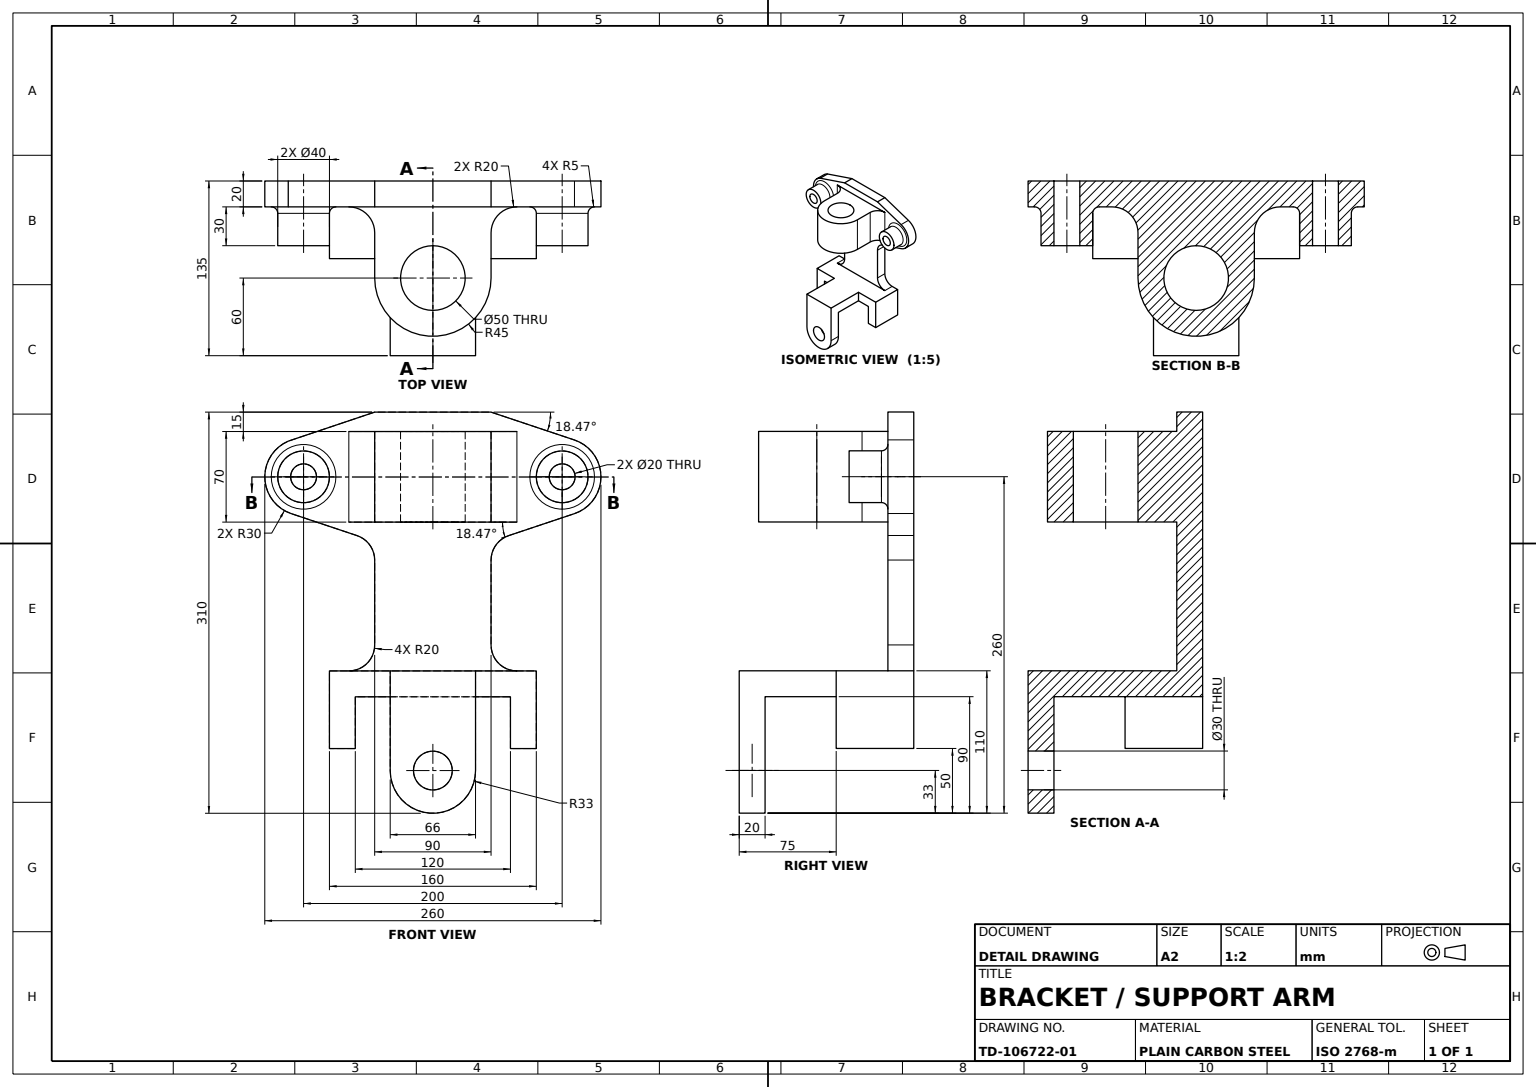
solid
v1 (-45,260,0)
v2 (-111.862968,237.554854,0)
e1 v1 v2 LINE
v3 (-111.862968,237.554854,20)
e2 v2 v3 LINE
v4 (-45,260,20)
e3 v4 v3 LINE
e4 v1 v4 LINE
face PLANE(AX(P(-45,260,0),D(-0.318236717,0.948011283,0),D(-0.948011283,-0.318236717,0))) [e1 e2 -e3 -e4]
v5 (109.504259,181.545316,20)
v6 (130,210,20)
e5 v5 v6 CIRCLE(AX(P(100,210,20),D(0,0,1),D(1,0,0)),30)
v7 (109.504259,181.545316,0)
e6 v7 v5 LINE
v8 (130,210,0)
e7 v7 v8 CIRCLE(AX(P(100,210,0),D(0,0,1),D(1,0,0)),30)
e8 v8 v6 LINE
face CYL(AX(P(100,210,0),D(0,0,1),D(1,0,0)),30) [-e5 -e6 e7 e8]
v9 (-75,210,20)
v10 (-125,210,20)
e9 v9 v10 CIRCLE(AX(P(-100,210,20),D(0,0,-1),D(-1,0,0)),25)
e10 v10 v9 CIRCLE(AX(P(-100,210,20),D(0,0,-1),D(-1,0,0)),25)
v11 (65,245,20)
v12 (-65,245,20)
e11 v11 v12 LINE
v13 (65,175,20)
e12 v11 v13 LINE
v14 (-65,175,20)
e13 v13 v14 LINE
e14 v14 v12 LINE
v15 (125,210,20)
v16 (75,210,20)
e15 v15 v16 CIRCLE(AX(P(100,210,20),D(0,0,-1),D(-1,0,0)),25)
e16 v16 v15 CIRCLE(AX(P(100,210,20),D(0,0,-1),D(-1,0,0)),25)
v17 (-58.663828,164.563908,20)
v18 (-45,145.594118,20)
e17 v17 v18 CIRCLE(AX(P(-65,145.594118,20),D(0,0,-1),D(-1,0,0)),20)
v19 (-45,80,20)
e18 v19 v18 LINE
v20 (-65,60,20)
e19 v19 v20 CIRCLE(AX(P(-65,80,20),D(0,0,-1),D(-1,0,0)),20)
v21 (65,60,20)
e20 v21 v20 LINE
v22 (45,80,20)
e21 v21 v22 CIRCLE(AX(P(65,80,20),D(0,0,-1),D(-1,0,0)),20)
v23 (45,145.594118,20)
e22 v23 v22 LINE
v24 (58.663828,164.563908,20)
e23 v23 v24 CIRCLE(AX(P(65,145.594118,20),D(0,0,-1),D(-1,0,0)),20)
e24 v24 v5 LINE
v25 (109.504259,238.454684,20)
e25 v6 v25 CIRCLE(AX(P(100,210,20),D(0,0,1),D(1,0,0)),30)
v26 (45,260,20)
e26 v25 v26 LINE
e27 v26 v4 LINE
v27 (-109.504259,181.545316,20)
e28 v3 v27 CIRCLE(AX(P(-100,210,20),D(0,0,1),D(1,0,0)),30)
e29 v27 v17 LINE
face PLANE(AX(P(0,0,20),D(0,0,-1),D(-1,0,0))) rev [e9 e10] [-e11 e12 e13 e14] [e15 e16] [e17 -e18 e19 -e20 e21 -e22 e23 e24 e5 e25 e26 e27 e3 e28 e29]
v28 (45,260,0)
e30 v28 v26 LINE
e31 v28 v1 LINE
face PLANE(AX(P(0,260,0),D(0,1,0),D(0,0,1))) [-e27 -e30 e31 e4]
v29 (-109.504259,181.545316,0)
e32 v29 v27 LINE
v30 (-58.663828,164.563908,0)
e33 v29 v30 LINE
e34 v30 v17 LINE
face PLANE(AX(P(-109.504259,181.545316,0),D(-0.31680862,-0.948489482,0),D(0.948489482,-0.31680862,0))) [-e29 -e32 e33 e34]
v31 (-120,210,25)
v32 (-80,210,25)
e35 v31 v32 CIRCLE(AX(P(-100,210,25),D(0,0,1),D(-1,0,0)),20)
v33 (-80,210,50)
e36 v33 v32 LINE
v34 (-120,210,50)
e37 v34 v33 CIRCLE(AX(P(-100,210,50),D(0,0,1),D(1,0,0)),20)
e38 v34 v31 LINE
face CYL(AX(P(-100,210,50),D(0,0,-1),D(-1,0,0)),20) [e35 -e36 -e37 e38]
v35 (90,210,50)
v36 (110,210,50)
e39 v35 v36 CIRCLE(AX(P(100,210,50),D(0,0,1),D(1,0,0)),10)
v37 (110,210,0)
e40 v37 v36 LINE
v38 (90,210,0)
e41 v38 v37 CIRCLE(AX(P(100,210,0),D(0,0,1),D(1,0,0)),10)
e42 v38 v35 LINE
face CYL(AX(P(100,210,-32),D(0,0,1),D(1,0,0)),10) rev [e39 -e40 -e41 e42]
v39 (15,-17,135)
v40 (-15,-17,135)
e43 v39 v40 CIRCLE(AX(P(0,-17,135),D(0,0,1),D(1,0,0)),15)
v41 (-15,-17,115)
e44 v41 v40 LINE
v42 (15,-17,115)
e45 v42 v41 CIRCLE(AX(P(0,-17,115),D(0,0,1),D(1,0,0)),15)
e46 v42 v39 LINE
face CYL(AX(P(0,-17,-80),D(0,0,1),D(1,0,0)),15) rev [e43 -e44 -e45 e46]
v43 (-60,40,60)
v44 (-60,40,0)
e47 v43 v44 LINE
v45 (-60,0,60)
e48 v45 v43 LINE
v46 (-60,0,0)
e49 v45 v46 LINE
e50 v46 v44 LINE
face PLANE(AX(P(-60,0,60),D(-1,0,0),D(0,0,1))) rev [-e47 -e48 e49 e50]
v47 (60,0,60)
v48 (80,0,60)
e51 v47 v48 LINE
v49 (60,0,0)
e52 v47 v49 LINE
v50 (80,0,0)
e53 v49 v50 LINE
e54 v48 v50 LINE
face PLANE(AX(P(60,0,60),D(0,1,0),D(0,0,1))) rev [-e51 e52 e53 -e54]
v51 (-33,-17,115)
v52 (-33,-17,135)
e55 v51 v52 LINE
v53 (33,-17,115)
e56 v51 v53 CIRCLE(AX(P(0,-17,115),D(0,0,1),D(1,0,0)),33)
v54 (33,-17,135)
e57 v53 v54 LINE
e58 v52 v54 CIRCLE(AX(P(0,-17,135),D(0,0,1),D(1,0,0)),33)
face CYL(AX(P(0,-17,115),D(0,0,1),D(1,0,0)),33) [-e55 e56 e57 -e58]
v55 (-90,210,0)
v56 (-90,210,50)
e59 v55 v56 LINE
v57 (-110,210,0)
e60 v57 v55 CIRCLE(AX(P(-100,210,0),D(0,0,1),D(1,0,0)),10)
v58 (-110,210,50)
e61 v57 v58 LINE
e62 v58 v56 CIRCLE(AX(P(-100,210,50),D(0,0,1),D(1,0,0)),10)
face CYL(AX(P(-100,210,-32),D(0,0,1),D(1,0,0)),10) rev [-e59 -e60 e61 e62]
e63 v32 v31 CIRCLE(AX(P(-100,210,25),D(0,0,1),D(-1,0,0)),20)
e64 v33 v34 CIRCLE(AX(P(-100,210,50),D(0,0,1),D(1,0,0)),20)
face CYL(AX(P(-100,210,50),D(0,0,-1),D(-1,0,0)),20) [e63 -e38 -e64 e36]
v59 (-80,0,60)
e65 v59 v45 LINE
v60 (-80,0,0)
e66 v59 v60 LINE
e67 v60 v46 LINE
face PLANE(AX(P(-80,0,60),D(0,1,0),D(0,0,1))) rev [-e65 e66 e67 -e49]
e68 v41 v42 CIRCLE(AX(P(0,-17,115),D(0,0,1),D(1,0,0)),15)
e69 v40 v39 CIRCLE(AX(P(0,-17,135),D(0,0,1),D(1,0,0)),15)
face CYL(AX(P(0,-17,-80),D(0,0,1),D(1,0,0)),15) rev [-e46 -e68 e44 e69]
v61 (60,40,60)
e70 v61 v47 LINE
v62 (60,40,0)
e71 v61 v62 LINE
e72 v62 v49 LINE
face PLANE(AX(P(60,40,60),D(1,0,0),D(0,0,-1))) rev [-e70 e71 e72 -e52]
v63 (45,80,0)
e73 v22 v63 LINE
v64 (45,145.594118,0)
e74 v64 v63 LINE
e75 v64 v23 LINE
face PLANE(AX(P(45,160,20),D(1,0,0),D(0,0,-1))) [e73 -e74 e75 e22]
v65 (65,60,0)
e76 v65 v21 LINE
e77 v63 v65 CIRCLE(AX(P(65,80,0),D(0,0,1),D(1,0,0)),20)
face CYL(AX(P(65,80,20),D(0,0,-1),D(-1,0,0)),20) rev [-e73 -e21 -e76 -e77]
v66 (-45,245,75)
v67 (-45,175,75)
e78 v66 v67 LINE
v68 (45,175,75)
e79 v67 v68 CIRCLE(AX(P(0,175,75),D(0,1,0),D(0,0,1)),45)
v69 (45,245,75)
e80 v69 v68 LINE
e81 v66 v69 CIRCLE(AX(P(0,245,75),D(0,1,0),D(0,0,1)),45)
face CYL(AX(P(0,245,75),D(0,-1,0),D(0,0,-1)),45) [e78 e79 -e80 -e81]
v70 (0,175,100)
v71 (0,245,100)
e82 v70 v71 LINE
v72 (0,175,50)
e83 v72 v70 CIRCLE(AX(P(0,175,75),D(0,1,0),D(0,0,1)),25)
v73 (0,245,50)
e84 v72 v73 LINE
e85 v73 v71 CIRCLE(AX(P(0,245,75),D(0,1,0),D(0,0,1)),25)
face CYL(AX(P(0,163,75),D(0,1,0),D(0,0,1)),25) rev [-e82 -e83 e84 e85]
e86 v56 v58 CIRCLE(AX(P(-100,210,50),D(0,0,1),D(1,0,0)),10)
e87 v55 v57 CIRCLE(AX(P(-100,210,0),D(0,0,1),D(1,0,0)),10)
face CYL(AX(P(-100,210,-32),D(0,0,1),D(1,0,0)),10) rev [e86 -e61 -e87 e59]
v74 (-45,145.594118,0)
e88 v18 v74 LINE
v75 (-45,80,0)
e89 v75 v74 LINE
e90 v75 v19 LINE
face PLANE(AX(P(-45,60,20),D(-1,0,0),D(0,0,1))) [e18 e88 -e89 e90]
e91 v70 v72 CIRCLE(AX(P(0,175,75),D(0,1,0),D(0,0,1)),25)
e92 v71 v73 CIRCLE(AX(P(0,245,75),D(0,1,0),D(0,0,1)),25)
face CYL(AX(P(0,163,75),D(0,1,0),D(0,0,1)),25) rev [-e84 -e91 e82 e92]
e93 v9 v32 CIRCLE(AX(P(-75,210,25),D(0,1,0),D(-1,0,0)),5)
e94 v10 v31 CIRCLE(AX(P(-125,210,25),D(0,-1,0),D(0,0,-1)),5)
face TORUS(AX(P(-100,210,25),D(0,0,-1),D(-1,0,0)),25,5) rev [-e93 -e10 e94 -e63]
v76 (-65,60,0)
e95 v76 v75 CIRCLE(AX(P(-65,80,0),D(0,0,1),D(1,0,0)),20)
e96 v20 v76 LINE
face CYL(AX(P(-65,80,60),D(0,0,-1),D(-1,0,0)),20) rev [-e90 -e95 -e96 -e19]
v77 (33,40,60)
e97 v77 v61 LINE
v78 (33,40,115)
e98 v78 v77 LINE
v79 (-33,40,115)
e99 v78 v79 LINE
v80 (-33,40,60)
e100 v80 v79 LINE
e101 v43 v80 LINE
e102 v44 v62 LINE
face PLANE(AX(P(-60,40,60),D(0,1,0),D(0,0,1))) rev [-e97 -e98 e99 -e100 -e101 e47 e102 -e71]
v81 (45,245,40)
e103 v69 v81 LINE
v82 (45,175,40)
e104 v68 v82 LINE
e105 v82 v81 LINE
face PLANE(AX(P(45,245,20),D(-1,0,0),D(0,0,1))) rev [-e103 e80 e104 e105]
face TORUS(AX(P(-100,210,25),D(0,0,-1),D(-1,0,0)),25,5) rev [-e9 e93 -e35 -e94]
v83 (120,210,25)
e106 v15 v83 CIRCLE(AX(P(125,210,25),D(0,1,0),D(-1,0,0)),5)
v84 (80,210,25)
e107 v84 v83 CIRCLE(AX(P(100,210,25),D(0,0,1),D(-1,0,0)),20)
e108 v16 v84 CIRCLE(AX(P(75,210,25),D(0,-1,0),D(0,0,-1)),5)
face TORUS(AX(P(100,210,25),D(0,0,-1),D(-1,0,0)),25,5) rev [e106 -e107 -e108 -e15]
v85 (-80,60,60)
e109 v85 v59 LINE
v86 (-80,60,0)
e110 v85 v86 LINE
e111 v86 v60 LINE
face PLANE(AX(P(-80,60,60),D(1,0,0),D(0,0,-1))) rev [-e109 e110 e111 -e66]
e112 v81 v11 CIRCLE(AX(P(65,245,40),D(0,-1,0),D(0,0,1)),20)
e113 v13 v82 CIRCLE(AX(P(65,175,40),D(0,1,0),D(0,0,1)),20)
face CYL(AX(P(65,0,40),D(0,1,0),D(0,0,1)),20) rev [-e112 -e105 -e113 -e12]
e114 v83 v84 CIRCLE(AX(P(100,210,25),D(0,0,1),D(-1,0,0)),20)
v87 (80,210,50)
e115 v87 v84 LINE
v88 (120,210,50)
e116 v88 v87 CIRCLE(AX(P(100,210,50),D(0,0,1),D(1,0,0)),20)
e117 v88 v83 LINE
face CYL(AX(P(100,210,50),D(0,0,-1),D(-1,0,0)),20) [e114 -e115 -e116 e117]
e118 v74 v30 CIRCLE(AX(P(-65,145.594118,0),D(0,0,1),D(1,0,0)),20)
face CYL(AX(P(-65,145.594118,20),D(0,0,1),D(1,0,0)),20) rev [-e118 -e88 -e17 -e34]
v89 (-45,245,40)
v90 (-45,175,40)
e119 v89 v90 LINE
e120 v90 v67 LINE
e121 v89 v66 LINE
face PLANE(AX(P(-45,245,75),D(1,0,0),D(0,0,-1))) rev [e119 e120 -e78 -e121]
e122 v36 v35 CIRCLE(AX(P(100,210,50),D(0,0,1),D(1,0,0)),10)
e123 v87 v88 CIRCLE(AX(P(100,210,50),D(0,0,1),D(1,0,0)),20)
face PLANE(AX(P(100,210,50),D(0,0,1),D(1,0,0))) [-e122 -e39] [e116 e123]
v91 (33,60,135)
e124 v54 v91 LINE
v92 (-33,60,135)
e125 v92 v91 LINE
e126 v52 v92 LINE
face PLANE(AX(P(0,40,135),D(0,0,1),D(1,0,0))) [e58 e124 -e125 -e126] [-e69 -e43]
v93 (109.504259,238.454684,0)
e127 v8 v93 CIRCLE(AX(P(100,210,0),D(0,0,1),D(1,0,0)),30)
e128 v93 v25 LINE
face CYL(AX(P(100,210,0),D(0,0,1),D(1,0,0)),30) [-e25 -e8 e127 e128]
v94 (58.663828,164.563908,0)
e129 v24 v94 LINE
e130 v94 v7 LINE
face PLANE(AX(P(109.504259,181.545316,0),D(0.31680862,-0.948489482,0),D(0.948489482,0.31680862,0))) [e6 -e24 e129 e130]
e131 v90 v14 CIRCLE(AX(P(-65,175,40),D(0,1,0),D(0,0,1)),20)
face PLANE(AX(P(0,175,75),D(0,1,0),D(0,0,1))) rev [-e13 e113 -e104 -e79 -e120 e131] [e83 e91]
v95 (-33,60,60)
e132 v95 v85 LINE
e133 v80 v95 LINE
face PLANE(AX(P(0,0,60),D(0,0,1),D(1,0,0))) [e132 e109 e65 e48 e101 e133]
e134 v12 v89 CIRCLE(AX(P(-65,245,40),D(0,-1,0),D(0,0,1)),20)
face PLANE(AX(P(0,245,75),D(0,1,0),D(0,0,1))) [e121 e81 e103 e112 e11 e134] [-e92 -e85]
e135 v93 v28 LINE
face PLANE(AX(P(45,260,0),D(0.31680862,0.948489482,0),D(-0.948489482,0.31680862,0))) [-e26 -e128 e135 e30]
face CYL(AX(P(-65,245,40),D(0,1,0),D(0,0,1)),20) rev [-e131 -e119 -e134 -e14]
e136 v94 v64 CIRCLE(AX(P(65,145.594118,0),D(0,0,1),D(1,0,0)),20)
face CYL(AX(P(65,145.594118,0),D(0,0,1),D(1,0,0)),20) rev [-e129 -e23 -e75 -e136]
v96 (33,60,60)
e137 v77 v96 LINE
e138 v91 v96 LINE
e139 v53 v78 LINE
face PLANE(AX(P(33,40,135),D(1,0,0),D(0,1,0))) [e98 e137 -e138 -e124 -e57 e139]
e140 v37 v38 CIRCLE(AX(P(100,210,0),D(0,0,1),D(1,0,0)),10)
v97 (80,60,0)
e141 v97 v65 LINE
e142 v50 v97 LINE
e143 v76 v86 LINE
e144 v2 v29 CIRCLE(AX(P(-100,210,0),D(0,0,1),D(1,0,0)),30)
face PLANE(AX(P(0,0,0),D(0,0,1),D(1,0,0))) rev [e87 e60] [e140 e41] [-e141 -e142 -e53 -e72 -e102 -e50 -e67 -e111 -e143 e95 e89 e118 -e33 -e144 -e1 -e31 -e135 -e127 -e7 -e130 e136 e74 e77]
face PLANE(AX(P(-100,210,50),D(0,0,1),D(1,0,0))) [e37 e64] [-e86 -e62]
e145 v95 v92 LINE
e146 v79 v51 LINE
face PLANE(AX(P(-33,40,60),D(-1,0,0),D(0,-1,0))) [-e145 -e133 e100 e146 e55 e126]
face CYL(AX(P(100,210,-32),D(0,0,1),D(1,0,0)),10) rev [-e42 -e140 e40 e122]
face TORUS(AX(P(100,210,25),D(0,0,-1),D(-1,0,0)),25,5) rev [-e114 -e106 -e16 e108]
face CYL(AX(P(-100,210,0),D(0,0,1),D(1,0,0)),30) [-e28 -e2 e144 e32]
face PLANE(AX(P(0,-17,115),D(0,0,1),D(1,0,0))) rev [-e99 -e139 -e56 -e146] [e45 e68]
v98 (80,60,60)
e147 v48 v98 LINE
e148 v98 v96 LINE
face PLANE(AX(P(0,0,60),D(0,0,1),D(1,0,0))) [e70 e51 e147 e148 -e137 e97]
e149 v98 v97 LINE
face PLANE(AX(P(80,60,60),D(0,-1,0),D(1,0,0))) rev [e96 e143 -e110 -e132 e145 e125 e138 -e148 e149 e141 e76 e20]
face PLANE(AX(P(80,0,60),D(-1,0,0),D(0,0,1))) rev [-e147 e54 e142 -e149]
face CYL(AX(P(100,210,50),D(0,0,-1),D(-1,0,0)),20) [-e123 e115 e107 -e117]
